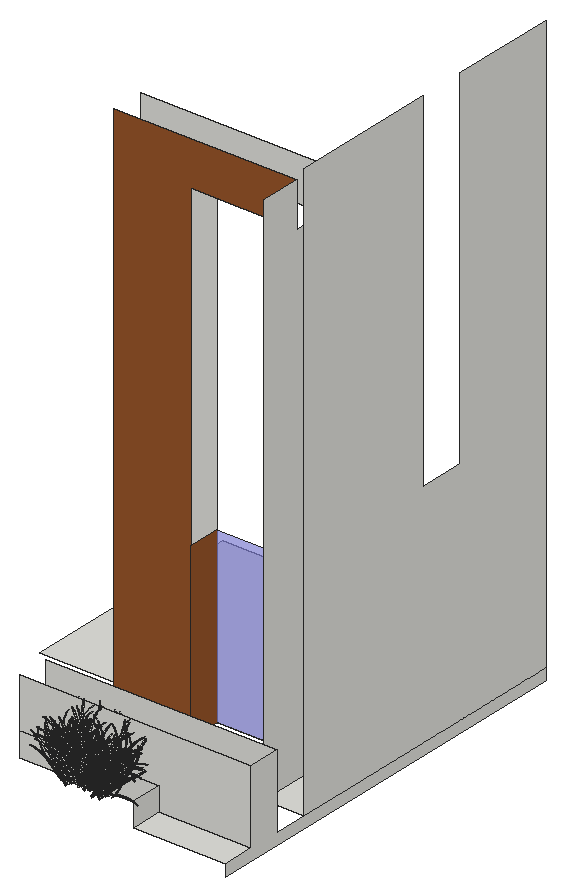
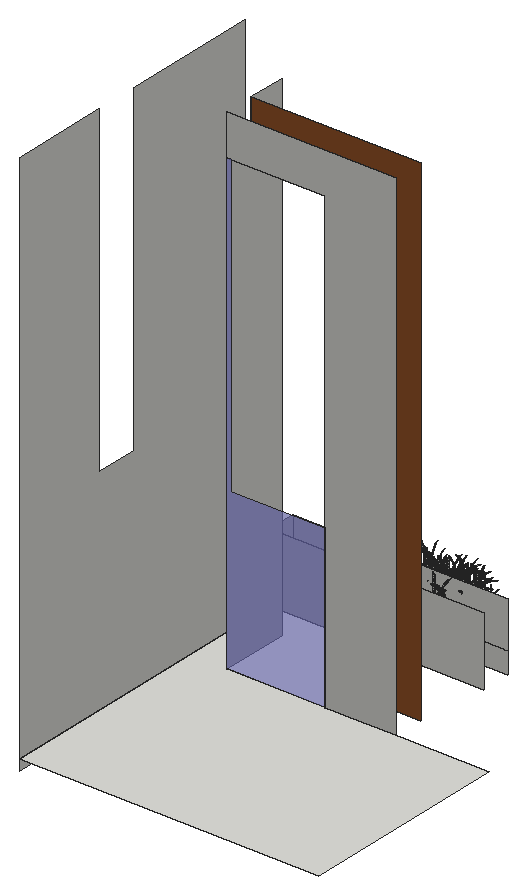
# SketchUp Ruby script. Lengths in inches.
U = 1.inch
M = Sketchup.active_model
def pt(a) = Geom::Point3d.new(a.map { |v| v * U })
def face(e, loops, mat)
  f = e.add_face(loops[0].map { |a| pt(a) })
  loops[1..].each { |l| e.add_face(l.map { |a| pt(a) }).erase! }
  f.material = f.back_material = mat if mat
  f
end
# faces: each face lists its corners as indices into pts; further lists are holes
def faces(e, pts, list, mat = nil) = list.each { |f| face(e, (f[0].is_a?(Array) ? f : [f]).map { |l| l.map { |i| pts[i] } }, mat) }
# xy, xz, yz: faces in a plane at the given z, y or x. An outline is a flat list of corners, or four numbers for a rectangle; further outlines are holes
def ring(l) = l.size == 4 ? [[l[0], l[1]], [l[2], l[1]], [l[2], l[3]], [l[0], l[3]]] : l.each_slice(2).to_a
def flat(e, list, mat, &to3) = list.each { |f| face(e, (f[0].is_a?(Array) ? f : [f]).map { |l| ring(l).map { |u, v| to3.(u, v) } }, mat) }
def xy(e, z, list, mat = nil) = flat(e, list, mat) { |x, y| [x, y, z] }
def xz(e, y, list, mat = nil) = flat(e, list, mat) { |x, z| [x, y, z] }
def yz(e, x, list, mat = nil) = flat(e, list, mat) { |y, z| [x, y, z] }
def lines(e, pts, list) = list.each { |a, b| e.add_line(pt(pts[a]), pt(pts[b])) }
# prism: a flat outline (further loops are holes) pulled along v
def prism(e, loops, v, mat = nil)
  f = face(e, loops, mat); d = Geom::Vector3d.new(v.map { |x| x * U })
  f.pushpull(f.normal.samedirection?(d) ? d.length : -d.length)
end
def box(e, o, s, mat = nil) = prism(e, [[o, [o[0] + s[0], o[1], o[2]], [o[0] + s[0], o[1] + s[1], o[2]], [o[0], o[1] + s[1], o[2]]]], [0, 0, s[2]], mat)
def at(x, y, z, deg = 0) = Geom::Transformation.translation(pt([x, y, z])) * Geom::Transformation.rotation(ORIGIN, Z_AXIS, deg.degrees)
def axes(o, x, y, z) = Geom::Transformation.new([*x, 0, *y, 0, *z, 0, *pt(o).to_a, 1])
def part(name) = M.definitions.add(name)
# library, detail: a bought-in or finely detailed component or shape, given as its bounding box
def library(name, o, s) = part(name).tap { |d| box(d.entities, o, s) }
def detail(e, o, s) = box(e.add_group.entities, o, s)
def put(e, d, t, mat = nil) = e.add_instance(d, t).tap { |i| i.material = mat if mat }
def group(e, t, mat = nil) = e.add_group.tap { |g| g.transformation = t; g.material = mat if mat }.entities
root = M.entities
M.materials.add("[Color I02]1").color = [153, 153, 255]
M.materials["[Color I02]1"].alpha = 0.68
M.materials.add("[Wood Cherry Original]").color = [152, 86, 42]
c1 = part("fur_instance\#8")
p = [[-0.25,1.49,0.03],[0.25,-1.49,-0.03],[0.44,-1.47,1.51],[-0.05,1.47,1.57],[0.65,-1.44,3.05],[0.16,1.45,3.11],
  [0.86,-1.42,4.59],[0.38,1.44,4.65],[1.1,-1.39,6.13],[0.62,1.43,6.18],[1.34,-1.35,7.66],[0.875,1.42,7.72],
  [1.6,-1.32,9.19],[1.14,1.41,9.25],[1.88,-1.28,10.72],[1.43,1.41,10.78],[2.18,-1.24,12.25],[1.73,1.41,12.3],
  [2.49,-1.19,13.77],[2.05,1.41,13.82],[2.83,-1.15,15.29],[2.4,1.41,15.34],[3.18,-1.09,16.8],[2.76,1.42,16.85],
  [3.56,-1.03,18.31],[3.14,1.43,18.35],[3.96,-0.97,19.81],[3.55,1.44,19.85],[4.38,-0.91,21.3],[3.99,1.46,21.35],
  [4.84,-0.83,22.78],[4.45,1.48,22.83],[5.32,-0.76,24.26],[4.93,1.51,24.31],[5.82,-0.67,25.73],[5.45,1.54,25.77],
  [6.36,-0.59,27.18],[6,1.57,27.23],[6.93,-0.49,28.625],[6.58,1.61,28.67],[7.54,-0.39,30.05],[7.19,1.66,30.1],
  [8.18,-0.28,31.47],[7.84,1.71,31.51],[8.85,-0.16,32.86],[8.53,1.77,32.9],[9.57,-0.04,34.24],[9.25,1.83,34.27],
  [10.32,0.09,35.59],[10.02,1.9,35.625],[11.12,0.23,36.92],[10.82,1.97,36.95],[11.95,0.38,38.22],[11.67,2.06,38.25],
  [12.84,0.54,39.49],[12.57,2.14,39.52],[13.76,0.71,40.73],[13.51,2.24,40.76],[14.73,0.89,41.93],[14.49,2.34,41.95],
  [15.75,1.08,43.09],[15.52,2.45,43.11],[16.82,1.28,44.2],[16.6,2.5625,44.23],[17.93,1.5,45.27],[17.73,2.68,45.29],
  [19.08,1.73,46.28],[18.9,2.81,46.3],[20.29,1.97,47.24],[20.125,2.93,47.26],[21.53,2.22,48.13],[21.39,3.0625,48.15],
  [22.82,2.5,48.96],[22.7,3.1875,48.98],[24.14,2.8125,49.72],[24.06,3.3,49.73],[25.48,3.27,50.41]]
faces(c1.entities,p,[[0,1,2,3],[3,2,4,5],[5,4,6,7],[7,6,8,9],[9,8,10,11],[11,10,12,13],[13,12,14,15],[15,14,16,17],
  [17,16,18,19],[19,18,20,21],[21,20,22,23],[23,22,24,25],[25,24,26,27],[27,26,28,29],[29,28,30,31],[31,30,32,33],
  [33,32,34,35],[35,34,36,37],[37,36,38,39],[39,38,40,41],[41,40,42,43],[43,42,44,45],[45,44,46,47],[47,46,48,49],
  [49,48,50,51],[51,50,52,53],[53,52,54,55],[55,54,56,57],[57,56,58,59],[59,58,60,61],[61,60,62,63],[63,62,64,65],
  [65,64,66,67],[67,66,68,69],[69,68,70,71],[71,70,72,73],[73,72,74,75],[75,74,76]])
xy(root,0,[[324.83,32.99,373.22,49.71],[352.27,84.18,352.27,122.8,204.07,122.8,204.07,242.8,373.22,242.8,373.22,84.18]])
xz(root,49.71,[[252.01,0,324.83,12.375],[324.83,0,373.22,0,373.22,38.6875,252.01,38.6875,252.01,12.375,324.83,12.375]])
xz(root,66.43,[[252.01,0,373.22,38.6875]])
xz(root,105.55,[[256.63,0,296.76,0,296.76,258.95,352.27,258.95,352.27,282.04,256.63,282.04]],"[Wood Cherry Original]")
xz(root,122.8,[[256.63,0,256.63,282.04,352.27,282.04,352.27,258.95,296.76,258.95,296.76,0]])
xz(root,122.8,[[296.76,0,352.27,0,352.27,258.95,349.59,258.95,349.59,90.8125,296.76,90.8125]],"[Color I02]1")
yz(root,296.76,[[105.55,0,122.8,90.8125]],"[Wood Cherry Original]")
yz(root,324.83,[[32.99,0,49.71,12.375]])
yz(root,352.27,[[84.18,0,84.18,282.04,105.55,282.04,105.55,258.95,122.8,258.95,122.8,0]])
yz(root,373.22,[[32.99,-6,242.8,-6,242.8,0,66.43,0,66.43,38.6875,49.71,38.6875,49.71,0,32.99,0],[84.18,0,242.8,0,242.8,304.31,186.78,304.31,186.78,120.43,162.34,120.43,162.34,304.31,84.18,304.31]])
put(root,c1,axes([297.07,29.66,14.5],[-0.37986,0.11496,-0.01734],[-0.11893,-0.25359,-0.04518],[-0.03923,-0.08677,0.40722]))
put(root,c1,axes([300.22,27.99,12.8],[-0.17462,0.20391,0.03429],[-0.27946,-0.10792,0.01354],[0.0209,-0.06883,0.33653]))
put(root,c1,axes([293.93,31.76,13.74],[-0.30043,-0.13979,-0.08203],[0.22786,-0.24984,0.08437],[-0.12286,-0.04065,0.38921]))
put(root,c1,axes([291.35,30.26,11.03],[0.27814,-0.07125,0.24103],[0.01578,0.25799,0.01434],[-0.24239,-0.02942,0.29163]))
put(root,c1,axes([309.31,30.78,9.9],[0.26005,-0.02253,-0.32035],[0.06182,0.2884,-0.05179],[0.3097,-0.0728,0.26576]))
put(root,c1,axes([306.62,31.4,9.98],[-0.12063,-0.20656,0.23753],[0.22477,-0.16177,-0.15489],[0.25439,0.01275,0.23669]))
put(root,c1,axes([300.89,28.39,13.19],[-0.00414,0.23821,0.05401],[-0.3412,-0.00346,0.09367],[0.08458,-0.09461,0.34384]))
put(root,c1,axes([292.09,29.77,9.76],[0.20353,-0.04601,0.26437],[-0.00599,0.23776,-0.01108],[-0.26313,-0.01442,0.2153]))
put(root,c1,axes([309.51,34.31,12.07],[-0.09639,-0.31824,0.12722],[0.35076,-0.08826,-0.26749],[0.27732,-0.04665,0.36362]))
put(root,c1,axes([298.73,28.3,13.26],[-0.08984,0.23712,0.03942],[-0.33625,-0.03634,-0.01926],[-0.01687,-0.08372,0.35457]))
put(root,c1,axes([302.43,31.45,14.3],[0.38172,-0.07813,-0.11304],[0.09285,0.27954,-0.03883],[0.10653,-0.06196,0.39986]))
put(root,c1,axes([302.73,28.04,12],[0.10021,0.21737,-0.04197],[-0.27272,0.07036,0.15178],[0.14611,-0.06349,0.29391]))
put(root,c1,axes([292.2,29.75,13.39],[-0.30752,0.22698,-0.0565],[-0.22359,-0.16067,-0.20167],[-0.1779,-0.12786,0.376]))
put(root,c1,axes([303.88,30.99,14.1],[0.39992,0.00155,-0.12267],[-0.00919,0.2918,0.01674],[0.11029,-0.07994,0.40704]))
put(root,c1,axes([295.86,30.04,13.95],[0.3361,0.0597,0.11647],[-0.14291,0.26481,-0.01688],[-0.12031,-0.07015,0.37628]))
put(root,c1,axes([314.07,32.9,10.36],[-0.31461,0.02837,0.40448],[-0.1367,-0.3405,0.01783],[0.37524,-0.14378,0.32832]))
put(root,c1,axes([298.375,28.95,14.06],[-0.23063,0.22567,0.03204],[-0.30414,-0.13521,-0.0359],[-0.0185,-0.09181,0.38884]))
put(root,c1,axes([290.27,32.23,9.95],[-0.02718,-0.26721,0.06111],[0.23487,-0.04018,0.2882],[-0.28708,0.02287,0.24209]))
put(root,c1,axes([305.03,31.13,9.43],[-0.06107,-0.20124,0.21197],[0.24192,-0.11583,-0.14036],[0.20685,0.04397,0.21399]))
put(root,c1,axes([294.54,31.76,12.14],[0.17245,-0.22481,0.15675],[0.27326,0.12505,0.06049],[-0.14508,0.02294,0.32196]))
put(root,c1,axes([295.24,33.11,14.17],[-0.1453,-0.26295,0.04416],[0.36594,-0.13308,0.10576],[-0.09136,-0.00185,0.39825]))
put(root,c1,axes([299.125,32.17,12.94],[-0.17065,-0.21754,0.08769],[0.31451,-0.14349,0.04448],[-0.00634,0.01342,0.35351]))
put(root,c1,axes([298.21,29.74,13.28],[0.32343,0.06667,0.01052],[-0.1253,0.24167,-0.02668],[-0.02751,-0.0389,0.35559]))
put(root,c1,axes([306.15,28.67,9.75],[-0.05331,0.21759,0.08334],[-0.21187,-0.0925,0.2518],[0.25313,-0.0595,0.21722]))
put(root,c1,axes([309.43,29.48,9.85],[0.01398,0.27039,0.10361],[-0.28188,-0.07693,0.31658],[0.30873,-0.11829,0.27013]))
put(root,c1,axes([295.78,30.16,12.95],[-0.33254,0.06855,-0.1047],[-0.04472,-0.24536,0.00177],[-0.10933,-0.03618,0.34634]))
put(root,c1,axes([299.96,30.99,13.19],[0.3311,-0.11143,-0.00818],[0.12332,0.23349,-0.09764],[0.03307,0.00434,0.3504]))
put(root,c1,axes([300.49,31.6,11.78],[0.12505,-0.22688,0.10637],[0.2992,0.06356,-0.10951],[0.05567,0.04516,0.30083]))
put(root,c1,axes([295.53,30.05,14.23],[0.26883,0.15362,0.11698],[-0.26881,0.22996,-0.03987],[-0.11858,-0.08853,0.38915]))
put(root,c1,axes([297.49,30.97,13.59],[-0.33593,-0.07204,-0.02348],[0.12579,-0.25592,0.09942],[-0.06598,0.00622,0.35973]))
put(root,c1,axes([300.72,29.6875,12.73],[0.31871,0.03853,-0.0833],[-0.07703,0.23988,-0.04321],[0.06207,-0.01348,0.32903]))
put(root,c1,axes([308.82,35.61,14.78],[0.22107,-0.31645,-0.08819],[0.39347,0.17405,-0.22486],[0.22281,-0.06522,0.45604]))
put(root,c1,axes([292.26,33,12.65],[-0.21857,-0.2084,-0.04599],[0.27515,-0.19846,0.18316],[-0.1798,0.00438,0.35795]))
put(root,c1,axes([299.6875,29.61,13.07],[0.27771,0.12403,-0.02683],[-0.1961,0.21075,-0.00493],[0.0103,-0.04126,0.34765]))
put(root,c1,axes([295.9375,29.46,12.93],[-0.25046,0.19218,-0.07567],[-0.21771,-0.16026,-0.07349],[-0.11089,-0.04968,0.34288]))
put(root,c1,axes([292.76,30.24,14.75],[-0.06283,0.2928,0.10996],[-0.40135,0.05052,-0.19489],[-0.19008,-0.13661,0.40174]))
put(root,c1,axes([305.98,30.41,12.04],[-0.21613,0.17279,0.19106],[-0.21553,-0.21071,0.16457],[0.23814,-0.07365,0.30654]))
put(root,c1,axes([299.64,33.21,13.75],[-0.22461,-0.21558,0.09909],[0.31674,-0.18353,0.03994],[0.01515,0.01113,0.38383]))
put(root,c1,axes([304.03,29.54,11.83],[-0.20447,0.18723,0.09128],[-0.23214,-0.16193,0.13811],[0.15272,-0.0447,0.31258]))
put(root,c1,axes([301.73,29.38,12.42],[0.25056,0.13748,-0.09261],[-0.20183,0.19585,0.01597],[0.07293,-0.02461,0.32493]))
put(root,c1,axes([293.94,30.14,13.9],[-0.26766,0.23648,-0.03819],[-0.2782,-0.15147,-0.11955],[-0.12042,-0.0899,0.39518]))
put(root,c1,axes([295.06,30.1875,12.98],[-0.31485,0.13604,-0.10356],[-0.13695,-0.22237,-0.02752],[-0.11187,-0.03702,0.3544]))
put(root,c1,axes([293.16,32.5625,11.3],[-0.03678,-0.25397,0.12997],[0.29931,-0.02143,0.19004],[-0.19333,0.05707,0.28615]))
put(root,c1,axes([304.64,31.96,13.24],[-0.36491,-0.01389,0.1859],[0.03737,-0.29294,0.04841],[0.16886,-0.0262,0.36677]))
put(root,c1,axes([296.76,30.3125,12.78],[-0.31334,0.10011,-0.09501],[-0.10112,-0.22757,0.02464],[-0.08992,-0.01108,0.3359]))
put(root,c1,axes([291.74,31.81,9.48],[0.14355,-0.1766,0.25684],[0.18766,0.16788,0.08409],[-0.24795,0.05471,0.22422]))
put(root,c1,axes([295.6,32.125,12.85],[-0.2833,-0.13793,-0.02305],[0.18987,-0.22311,0.16973],[-0.12695,0.04004,0.33147]))
put(root,c1,axes([291.51,30.93,13.19],[0.25521,0.1512,0.17452],[-0.25665,0.25153,-0.10558],[-0.20333,-0.07415,0.37359]))
put(root,c1,axes([298.13,31.5625,11.92],[-0.26729,-0.12063,0.06749],[0.18715,-0.19794,0.13627],[-0.03388,0.05903,0.30001]))
put(root,c1,axes([302.29,30.11,13.34],[0.22509,0.19991,-0.07599],[-0.27838,0.17319,0.07803],[0.09708,-0.05646,0.36438]))
put(root,c1,axes([304.44,30.18,12.87],[-0.10789,0.25373,0.07285],[-0.32713,-0.09482,0.17189],[0.17322,-0.07527,0.34846]))
put(root,c1,axes([301.9375,33.34,12.41],[-0.18573,-0.21093,0.17304],[0.30858,-0.16641,-0.00938],[0.0929,0.03699,0.33971]))
put(root,c1,axes([301.17,33.54,12.34],[0.02005,-0.26344,0.15335],[0.36284,-0.01782,-0.07584],[0.06238,0.05061,0.33711]))
put(root,c1,axes([302.27,33.05,14.28],[0.3894,-0.10534,-0.06303],[0.1122,0.28119,-0.09735],[0.07672,-0.01666,0.40666]))
put(root,c1,axes([304.9375,32.15,11.95],[0.31108,-0.11547,-0.14728],[0.08809,0.24884,-0.19208],[0.19555,0.02546,0.30249]))
put(root,c1,axes([310.28,36.01,13.41],[0.26375,-0.26825,-0.16948],[0.29485,0.23881,-0.27394],[0.30159,-0.05073,0.39544]))
put(root,c1,axes([305.46,33.45,11.4],[0.25076,-0.21435,-0.05395],[0.21574,0.18121,-0.2417],[0.20008,0.02605,0.30949]))
put(root,c1,axes([307.5,33.67,12.11],[0.30932,-0.16941,-0.1706],[0.16282,0.26082,-0.21532],[0.24459,-0.00639,0.3404]))
put(root,c1,axes([296.91,34.89,14.07],[-0.1186,-0.27751,0.08841],[0.38874,-0.1102,0.0715],[-0.0532,0.01296,0.40459]))
put(root,c1,axes([306.88,34.04,11.42],[-0.17025,-0.23312,0.23887],[0.30544,-0.18356,-0.10713],[0.2115,0.02754,0.32717]))
put(root,c1,axes([303.75,30.85,11.85],[-0.31518,0.08138,0.11458],[-0.07485,-0.24165,0.11876],[0.13173,-0.00126,0.31832]))
put(root,c1,axes([302.64,34.5625,16.18],[0.42095,-0.14725,-0.10442],[0.17691,0.30585,-0.08745],[0.1162,-0.05293,0.46349]))
put(root,c1,axes([292.29,31.73,12.13],[-0.32982,0.0527,-0.18032],[-0.01849,-0.26967,0.0269],[-0.1831,-0.01848,0.34164]))
put(root,c1,axes([294.35,32.48,11.32],[-0.17974,-0.20388,0.06604],[0.25023,-0.12836,0.21159],[-0.15875,0.07631,0.27776]))
put(root,c1,axes([288.31,31.25,10.58],[0.14971,0.15077,0.26268],[-0.21096,0.2535,-0.19987],[-0.32252,-0.06234,0.26598]))
put(root,c1,axes([297.09,29.33,12.93],[0.00143,0.24353,-0.03417],[-0.32321,0.03016,-0.09258],[-0.09858,-0.02214,0.33211]))
put(root,c1,axes([300.8,30.81,14.04],[0.32079,0.12524,-0.10886],[-0.18999,0.24738,0.00297],[0.08451,-0.02851,0.37652]))
put(root,c1,axes([287.89,32.19,11.4],[0.25708,0.10485,0.25987],[-0.20499,0.28763,-0.11391],[-0.27939,-0.07246,0.33941]))
put(root,c1,axes([295.05,32.47,13.86],[0.38017,-0.03428,0.09673],[0.00663,0.28506,-0.0591],[-0.10384,-0.01279,0.3879]))
put(root,c1,axes([304.9,35.46,13.89],[-0.21678,-0.25794,0.18892],[0.34901,-0.19506,-0.09005],[0.16707,-0.0016,0.40371]))
put(root,c1,axes([297.7,30.01,13.23],[-0.01029,0.24957,-0.01761],[-0.34619,0.0186,-0.02439],[-0.03281,-0.04143,0.35542]))
put(root,c1,axes([299.64,31.97,12.16],[-0.30501,-0.08008,0.0968],[0.14614,-0.2274,0.12372],[0.02756,0.05561,0.31043]))
put(root,c1,axes([297.65,32.28,14.4375],[-0.38282,0.09711,-0.02143],[-0.09773,-0.2685,0.02287],[-0.02447,-0.04231,0.40465]))
put(root,c1,axes([294.07,30.88,10.86],[0.25741,0.03344,0.16681],[-0.0417,0.2339,-0.12911],[-0.1963,0.02845,0.25979]))
put(root,c1,axes([299.35,30.33,13.14],[-0.29118,0.15292,-0.03089],[-0.18473,-0.19959,0.08971],[0.01345,0.00988,0.34087]))
put(root,c1,axes([296.21,30.16,13.16],[0.14937,0.21705,0.01001],[-0.30573,0.14011,-0.10341],[-0.10379,-0.02331,0.34963]))
put(root,c1,axes([299.28,30.3,13.45],[0.09139,0.24124,-0.02708],[-0.34395,0.08755,0.00024],[-0.00171,-0.03839,0.36389]))
put(root,c1,axes([292,30.13,11.09],[0.06312,0.2347,0.05533],[-0.26357,0.11274,-0.22829],[-0.2358,-0.02862,0.28371]))
put(root,c1,axes([301.01,29.86,12.8],[0.02445,0.24426,-0.06773],[-0.33257,0.03724,0.06724],[0.06313,-0.01371,0.33464]))
put(root,c1,axes([301.4375,33.59,16.1875],[0.44361,0.00954,-0.12956],[-0.03541,0.33069,-0.02892],[0.11325,-0.05159,0.45172]))
put(root,c1,axes([298.8125,30.33,12.92],[-0.24792,0.18255,-0.06135],[-0.23021,-0.1655,0.06985],[-0.00599,0.01269,0.33425]))
put(root,c1,axes([292.85,31.49,13.32],[0.22087,0.18128,0.12698],[-0.26546,0.22192,-0.14635],[-0.19746,-0.04494,0.3589]))
put(root,c1,axes([301.2,30.7,12.46],[-0.2311,0.19122,-0.01481],[-0.24074,-0.15447,0.09263],[0.04816,-0.00374,0.33273]))
put(root,c1,axes([307.89,32.19,14.26],[-0.10311,0.30987,0.12078],[-0.41871,-0.10394,0.20078],[0.20991,-0.12435,0.43231]))
put(root,c1,axes([299.71,32.49,11.62],[-0.31244,-0.05998,0.08505],[0.11859,-0.23055,0.12985],[0.02723,0.05495,0.30674]))
put(root,c1,axes([288.9375,33.78,11.8],[0.31888,-0.08776,0.27392],[0.0591,0.29525,-0.01943],[-0.27072,0.00273,0.33496]))
put(root,c1,axes([290.05,34.25,10.97],[0.26388,-0.16586,0.25638],[0.17817,0.23606,0.02465],[-0.23968,0.03474,0.31721]))
put(root,c1,axes([303.36,31.49,11.12],[0.28654,0.0293,-0.18535],[-0.09478,0.23872,-0.10787],[0.14833,0.04775,0.26999]))
put(root,c1,axes([306.97,32.19,13.47],[0.21529,0.26732,-0.1015],[-0.33179,0.15897,0.18881],[0.1989,-0.08642,0.4001]))
put(root,c1,axes([296.45,32.43,13.07],[0.34376,0.06003,0.02841],[-0.1102,0.26073,-0.0988],[-0.0664,0.00626,0.36202]))
put(root,c1,axes([307.04,31.4,11.7],[-0.10758,0.27316,0.04345],[-0.30064,-0.09702,0.25634],[0.24342,-0.04095,0.31917]))
put(root,c1,axes([294.3125,31.78,13.16],[-0.28482,0.16744,-0.17926],[-0.17967,-0.21914,-0.02481],[-0.1723,0.0042,0.34303]))
put(root,c1,axes([297.99,32.49,12.83],[0.3546,-0.04207,0.0418],[0.03679,0.24974,-0.16079],[-0.03701,0.06449,0.32778]))
put(root,c1,axes([303.89,30.28,11.28],[-0.00719,0.23917,-0.12291],[-0.2843,0.03205,0.17385],[0.17201,0.0224,0.26607]))
put(root,c1,axes([310.13,32.77,9.65],[-0.23743,0.1703,0.23472],[-0.15105,-0.25518,0.23763],[0.31546,-0.02981,0.27622]))
put(root,c1,axes([292.56,33.74,13.97],[-0.37552,0.02978,-0.18444],[-0.00274,-0.30609,0.08192],[-0.19214,0.00468,0.38253]))
put(root,c1,axes([301.625,32.89,11.47],[0.32327,-0.10712,-0.01749],[0.09339,0.2108,-0.21888],[0.08265,0.08899,0.27927]))
put(root,c1,axes([289.88,32.2,9.47],[0.22299,0.08012,0.23253],[-0.07774,0.25772,-0.18032],[-0.28674,0.02285,0.2418]))
put(root,c1,axes([299.68,31.02,13.39],[0.09517,0.24549,-0.09781],[-0.34506,0.0918,0.01689],[0.0335,0.00439,0.35498]))
put(root,c1,axes([298.21,35.625,12.82],[0.21798,-0.24571,0.14926],[0.32986,0.13334,-0.10586],[-0.00426,0.0705,0.36176]))
put(root,c1,axes([297.91,36.18,12.93],[0.12837,-0.2754,0.18421],[0.3803,0.07387,-0.03249],[-0.04167,0.07261,0.36905]))
put(root,c1,axes([292.99,32.01,10.625],[-0.21375,0.16044,-0.2188],[-0.17312,-0.19073,-0.04043],[-0.20706,0.03001,0.27404]))
put(root,c1,axes([296.8,36.26,12.95],[0.11216,-0.27982,0.18642],[0.38756,0.06205,-0.02451],[-0.04189,0.07299,0.37096]))
put(root,c1,axes([300.57,32.22,11.33],[-0.32555,0.01552,0.05629],[0.02551,-0.21913,0.2004],[0.03956,0.09625,0.26535]))
put(root,c1,axes([303.87,34.79,9.58],[-0.07713,-0.20181,0.27533],[0.31715,-0.12915,-0.06147],[0.15566,0.11006,0.24058]))
put(root,c1,axes([294.44,31.52,11.55],[0.10989,0.22592,-0.04424],[-0.2903,0.10013,-0.15522],[-0.13937,0.02203,0.30928]))
put(root,c1,axes([302.81,32.85,15.3125],[0.10532,0.30402,-0.04355],[-0.41529,0.08818,0.12286],[0.11618,-0.06757,0.43608]))
put(root,c1,axes([293.17,34.71,15.125],[-0.41497,0.11282,-0.12938],[-0.10014,-0.30383,0.01576],[-0.1302,-0.02924,0.43863]))
put(root,c1,axes([296.16,32.57,11.97],[0.30429,0.09538,0.01629],[-0.13866,0.22954,-0.16183],[-0.09588,0.05048,0.31741]))
put(root,c1,axes([292.96,34.11,9.71],[-0.28109,-0.11553,-0.06299],[0.09114,-0.20051,0.26985],[-0.19429,0.11376,0.23386]))
put(root,c1,axes([301.5,31.45,11.39],[-0.09337,0.22828,-0.11476],[-0.30505,-0.0402,0.09688],[0.05476,0.04443,0.29594]))
put(root,c1,axes([299.04,34.23,13.18],[0.3826,-0.06128,0.01902],[0.05373,0.26621,-0.17779],[-0.00416,0.06889,0.3535]))
put(root,c1,axes([296.6875,32.12,11.73],[-0.22053,0.18022,-0.15283],[-0.23513,-0.15794,0.03506],[-0.09243,0.04867,0.306]))
put(root,c1,axes([294.78,34.97,10.76],[0.2625,-0.14738,0.21205],[0.21669,0.19878,-0.09487],[-0.13116,0.09754,0.29312]))
put(root,c1,axes([295.42,33.2,10.49],[0.31269,0.01357,0.09328],[-0.00239,0.22692,-0.19194],[-0.12049,0.0896,0.26927]))
put(root,c1,axes([307.39,32.0625,9.94],[0.01192,0.2682,-0.15387],[-0.26672,0.05898,0.25379],[0.26625,0.01334,0.24773]))
put(root,c1,axes([294.62,33.49,10.86],[0.31025,0.02136,0.12942],[-0.00842,0.24175,-0.18196],[-0.15992,0.07687,0.2798]))
put(root,c1,axes([298.14,34.6875,10.125],[-0.03498,-0.20006,0.26264],[0.33857,-0.02028,0.05275],[-0.05072,0.15008,0.22962]))
put(root,c1,axes([304.75,33.74,11.91],[-0.34714,0.09005,0.13903],[-0.04585,-0.2641,0.20633],[0.17209,0.0554,0.31324]))
put(root,c1,axes([303.93,35.28,10.24],[0.30429,-0.17714,0.00045],[0.15067,0.17535,-0.29348],[0.16193,0.1145,0.25028]))
put(root,c1,axes([301.15,35.4,9.74],[0.02171,-0.21225,0.26978],[0.35113,-0.03257,-0.06302],[0.05505,0.14594,0.23778]))
put(root,c1,axes([304.93,33.43,14.19],[0.16792,0.28009,-0.14825],[-0.36004,0.14978,0.14596],[0.18288,-0.02838,0.39722]))
put(root,c1,axes([295.57,33.97,11.49],[0.33335,-0.01288,0.12248],[0.03512,0.24333,-0.19321],[-0.12916,0.09605,0.28864]))
put(root,c1,axes([298.59,34.16,14.93],[-0.36467,0.17722,-0.05568],[-0.21281,-0.2513,0.10179],[-0.00748,0.01584,0.41713]))
put(root,c1,axes([297.71,32.1,12.31],[0.07759,0.23448,-0.13461],[-0.3281,0.06649,-0.08615],[-0.06621,0.05797,0.31394]))
put(root,c1,axes([297.97,32.45,11.12],[0.26871,0.1121,-0.09185],[-0.17857,0.18234,-0.18441],[-0.04158,0.10221,0.26229]))
put(root,c1,axes([291.68,33.52,9.99],[-0.2282,0.09889,-0.27706],[-0.15507,-0.22815,0.06699],[-0.23524,0.08977,0.23863]))
put(root,c1,axes([303.21,36.85,11.17],[-0.22074,-0.19332,0.24763],[0.32228,-0.19488,0.06048],[0.09595,0.1033,0.32421]))
put(root,c1,axes([301.02,33.47,9.91],[-0.32142,0.01588,0.07582],[0.04323,-0.19732,0.24388],[0.05075,0.13454,0.2192]))
put(root,c1,axes([291.42,35.39,9.9],[0.25074,-0.08755,0.28619],[0.14655,0.24668,-0.09015],[-0.24763,0.0945,0.2512]))
put(root,c1,axes([301.02,34.29,13.54],[-0.37668,0.11666,0.0198],[-0.11531,-0.26137,0.1844],[0.06763,0.05486,0.36544]))
put(root,c1,axes([299.37,33.28,14.04],[-0.08791,0.28558,-0.09756],[-0.38541,-0.03903,0.04808],[0.01542,0.01133,0.39076]))
put(root,c1,axes([291.32,33.33,11.09],[-0.13915,0.24729,-0.20336],[-0.27037,-0.1215,-0.13837],[-0.2289,0.03317,0.30295]))
put(root,c1,axes([297.18,33.7,9.77],[-0.30471,0.02079,-0.10877],[-0.06538,-0.19372,0.22972],[-0.09578,0.13621,0.21711]))
put(root,c1,axes([307.42,34.21,10.3],[-0.29712,0.14734,0.1685],[-0.08067,-0.24572,0.26461],[0.25524,0.05426,0.26405]))
put(root,c1,axes([306.58,34.3,12.69],[0.2149,0.22877,-0.24278],[-0.27792,0.213,0.13148],[0.24582,-0.00643,0.34211]))
put(root,c1,axes([297.23,35.37,10.27],[0.21532,-0.16466,0.23481],[0.27912,0.12752,-0.1478],[-0.05253,0.15544,0.23782]))
put(root,c1,axes([304.37,34.36,11.59],[-0.32789,0.1435,0.09153],[-0.1181,-0.23778,0.2301],[0.17128,0.05514,0.31177]))
put(root,c1,axes([291.21,38.76,11.93],[0.03426,-0.30148,0.23803],[0.38836,0.04526,0.14837],[-0.20088,0.09657,0.35147]))
put(root,c1,axes([303.36,33.71,10.27],[-0.31347,0.1074,0.08336],[-0.04707,-0.20642,0.26099],[0.15117,0.10689,0.23365]))
put(root,c1,axes([304.01,33.1,10.39],[-0.22722,0.20575,-0.01496],[-0.18573,-0.12856,0.27335],[0.19083,0.07929,0.23211]))
put(root,c1,axes([300.94,34,11.25],[0.31948,0.06732,-0.13282],[-0.14912,0.22743,-0.18129],[0.04271,0.10392,0.2865]))
put(root,c1,axes([296.73,35.09,15.26],[0.34747,0.16946,-0.03102],[-0.25995,0.27004,-0.11737],[-0.05681,0.01384,0.43198]))
put(root,c1,axes([308.42,34.29,9.73],[-0.16741,0.26625,0.03865],[-0.23369,-0.12855,0.31721],[0.28667,0.01437,0.26672]))
put(root,c1,axes([290.1,35.47,14.55],[0.26115,0.22486,0.10659],[-0.3089,0.25028,-0.19615],[-0.22421,-0.02263,0.41834]))
put(root,c1,axes([294.53,33.1,10.75],[-0.0094,0.23776,-0.17948],[-0.3052,-0.02188,-0.12668],[-0.15733,0.07563,0.27528]))
put(root,c1,axes([289.83,37.49,11.28],[0.3275,-0.1168,0.26372],[0.15078,0.28145,-0.07889],[-0.23114,0.06823,0.34212]))
put(root,c1,axes([302.13,36.55,14.42],[0.42486,0.00795,-0.14048],[-0.06464,0.32048,-0.15173],[0.11085,0.04413,0.40535]))
put(root,c1,axes([302.29,34.15,12.1875],[-0.3135,0.16987,0.01114],[-0.167,-0.20326,0.24037],[0.13137,0.078,0.30476]))
put(root,c1,axes([295.39,36.1875,10.66],[0.33995,-0.08561,0.14528],[0.13056,0.23485,-0.18927],[-0.09324,0.11245,0.30268]))
put(root,c1,axes([293.92,34.72,11.03],[-0.27426,0.12888,-0.22321],[-0.18187,-0.22273,0.07892],[-0.16956,0.08151,0.29667]))
put(root,c1,axes([301.71,37.94,12.88],[0.34147,-0.21227,0.0692],[0.24226,0.20372,-0.26431],[0.10284,0.11072,0.34749]))
put(root,c1,axes([306.35,36.45,11.83],[0.37826,0.00458,-0.22144],[-0.08147,0.30831,-0.16295],[0.19016,0.06122,0.34614]))
put(root,c1,axes([304.49,36.6,11.29],[0.38407,-0.04972,-0.14005],[-0.0124,0.28223,-0.21944],[0.14212,0.08438,0.32969]))
put(root,c1,axes([306.7,37.35,10.33],[-0.2882,-0.08649,0.31541],[0.20824,-0.28093,0.1026],[0.2312,0.09606,0.28122]))
put(root,c1,axes([312.66,39.45,12.56],[-0.42715,-0.02419,0.32817],[0.06651,-0.38387,0.08793],[0.30249,-0.00791,0.42097]))
put(root,c1,axes([291.51,35.48,10.39],[0.29431,0.04362,0.2094],[0.00668,0.26171,-0.22058],[-0.251,0.09579,0.25462]))
put(root,c1,axes([300.52,36.84,12.89],[-0.41299,0.03386,0.04001],[-0.00291,-0.29245,0.18761],[0.03366,0.06791,0.37907]))
put(root,c1,axes([310.5,40.86,11.73],[-0.13778,-0.29005,0.35264],[0.36274,-0.21506,-0.17875],[0.32168,0.06838,0.33279]))
put(root,c1,axes([299.37,37.77,12.49],[0.33122,-0.18689,0.15289],[0.2535,0.20157,-0.21508],[-0.00144,0.13013,0.33652]))
put(root,c1,axes([308.93,34.72,9.85],[-0.00687,0.30102,-0.15108],[-0.29585,0.04507,0.29223],[0.29511,0.01479,0.27458]))
put(root,c1,axes([303.06,37.22,13.75],[-0.42743,0.07152,0.09854],[-0.04242,-0.31234,0.18166],[0.11079,0.04411,0.40514]))
put(root,c1,axes([307.03,41.19,12.63],[0.2599,-0.31873,0.06706],[0.35593,0.1475,-0.30589],[0.2166,0.06973,0.39426]))
put(root,c1,axes([302.15,33.85,11.16],[0.07213,0.22522,-0.22426],[-0.3401,0.09466,0.03435],[0.0854,0.09194,0.28855]))
put(root,c1,axes([295.42,34.38,11.47],[0.26352,0.16628,-0.05182],[-0.2153,0.18316,-0.22638],[-0.13112,0.09751,0.29304]))
put(root,c1,axes([298.42,37.23,13.28],[-0.42137,0.02708,0.0056],[-0.00179,-0.2967,0.19494],[-0.00454,0.07514,0.38554]))
put(root,c1,axes([295.73,34.89,12.68],[-0.22933,0.22711,-0.17211],[-0.30435,-0.15593,0.05487],[-0.07483,0.06553,0.35485]))
put(root,c1,axes([302.41,35.34,11.77],[-0.35266,0.13842,0.00001],[-0.13312,-0.22585,0.24598],[0.09259,0.09969,0.31285]))
put(root,c1,axes([302.54,36.24,10.17],[-0.34668,0.00002,0.16605],[0.10374,-0.23905,0.24417],[0.11321,0.13888,0.25286]))
put(root,c1,axes([296.6,36.59,11.17],[-0.3813,0.02071,-0.04148],[-0.01778,-0.25239,0.24019],[-0.04919,0.12092,0.31033]))
put(root,c1,axes([299.71,33.95,9.75],[-0.12599,0.1857,-0.23333],[-0.30463,-0.05364,0.10641],[0.00132,0.14289,0.22018]))
put(root,c1,axes([291.79,36.76,14.23],[-0.33372,0.20578,-0.21383],[-0.24038,-0.25468,0.00327],[-0.18466,0.0292,0.40979]))
put(root,c1,axes([295.15,35.625,15.47],[0.07852,0.31662,-0.09055],[-0.4353,0.08503,-0.08758],[-0.08136,0.00767,0.44358]))
put(root,c1,axes([288.92,37.31,11.92],[0.36947,0.05041,0.18865],[-0.04561,0.31057,-0.21258],[-0.23866,0.07045,0.35325]))
put(root,c1,axes([292.39,35.6,14.32],[0.01367,0.31876,-0.11898],[-0.40177,0.02856,-0.17186],[-0.1805,0.02854,0.40055]))
put(root,c1,axes([297.68,38.93,10.55],[0.07836,-0.23298,0.31495],[0.3945,0.04674,-0.03186],[-0.05994,0.17735,0.27135]))
put(root,c1,axes([294.41,34.6875,9.85],[0.21397,0.18598,-0.12116],[-0.23548,0.11646,-0.24718],[-0.15132,0.13358,0.23391]))
put(root,c1,axes([292.83,38.43,10],[0.26548,-0.13957,0.28848],[0.25342,0.21117,-0.13271],[-0.17456,0.15409,0.26982]))
put(root,c1,axes([305.96,39.49,10.09],[-0.25932,-0.14611,0.33128],[0.29947,-0.25143,0.08652],[0.18892,0.13358,0.29199]))
put(root,c1,axes([304.72,41.42,12.91],[0.35972,-0.25581,0.03582],[0.27505,0.22046,-0.30467],[0.16747,0.09944,0.38851]))
put(root,c1,axes([302.55,40.09,9.99],[-0.09732,-0.23155,0.33127],[0.39501,-0.13642,-0.02153],[0.12728,0.15613,0.28427]))
put(root,c1,axes([305.14,41.64,12.39],[-0.25869,-0.23017,0.30476],[0.36959,-0.24537,0.02287],[0.16684,0.09906,0.38705]))
put(root,c1,axes([306.95,35.87,10.84],[-0.11682,0.297,-0.11687],[-0.29865,-0.02915,0.30513],[0.26586,0.05652,0.27504]))
put(root,c1,axes([291.64,40,10.8125],[0.06295,-0.25616,0.33273],[0.38873,0.09023,0.07333],[-0.18729,0.16533,0.2895]))
put(root,c1,axes([292.7,35.6,10.28],[0.25121,0.18786,-0.0324],[-0.19191,0.16123,-0.29466],[-0.20785,0.1217,0.25018]))
put(root,c1,axes([300.36,36.91,15.48],[0.07458,0.32412,-0.12197],[-0.45103,0.08366,0.03458],[0.04279,0.00561,0.45337]))
put(root,c1,axes([291.96,39.58,14.48],[0.44422,0.0077,0.13813],[-0.02634,0.34217,-0.1757],[-0.16565,0.05224,0.43251]))
put(root,c1,axes([295.34,36.37,11.39],[-0.26525,0.17982,-0.21681],[-0.26655,-0.18517,0.11704],[-0.09629,0.11611,0.31256]))
put(root,c1,axes([298.34,36.66,10.54],[0.36323,0.03464,-0.08776],[-0.09991,0.21815,-0.27961],[0.00151,0.16329,0.25161]))
put(root,c1,axes([296.57,37.88,16.47],[-0.32829,0.27565,-0.11166],[-0.35147,-0.21756,0.07209],[-0.03602,0.01858,0.47629]))
put(root,c1,axes([306.02,36.02,9.94],[-0.05641,0.27329,-0.21756],[-0.32994,0.04346,0.22398],[0.21766,0.09043,0.26474]))
put(root,c1,axes([290.28,38,12.17],[0.30671,0.1858,0.0706],[-0.20831,0.25234,-0.27412],[-0.23769,0.07017,0.35181]))
put(root,c1,axes([290.9,37.84,10.74],[-0.2561,0.14005,-0.3145],[-0.23719,-0.23476,0.09074],[-0.22951,0.13438,0.27625]))
put(root,c1,axes([307.5625,38.53,14.88],[0.13241,0.34234,-0.18022],[-0.44893,0.13613,0.1561],[0.19033,-0.00183,0.45992]))
put(root,c1,axes([306.74,39.9375,10.8],[-0.37717,0.05337,0.25249],[0.05977,-0.31116,0.2513],[0.24832,0.10317,0.30203]))
put(root,c1,axes([295.35,38.03,12.52],[-0.33315,0.15868,-0.21082],[-0.23691,-0.23143,0.16521],[-0.10467,0.12623,0.33978]))
put(root,c1,axes([299.99,38.14,13.44],[-0.27152,0.26137,-0.12674],[-0.33932,-0.16629,0.15711],[0.03541,0.07146,0.39888]))
put(root,c1,axes([299.84,38.33,11.27],[0.33259,0.12189,-0.18697],[-0.23311,0.24454,-0.17908],[0.0492,0.11972,0.33005]))
put(root,c1,axes([295.4375,39.05,11.76],[-0.38715,0.08937,-0.158],[-0.13683,-0.26731,0.21776],[-0.10514,0.12679,0.3413]))
put(root,c1,axes([299.06,37.66,10.33],[-0.35896,0.1108,-0.10677],[-0.15016,-0.19943,0.28324],[0.00156,0.16866,0.25988]))
put(root,c1,axes([297.58,40.57,12.68],[-0.44662,-0.00971,0.04606],[0.05707,-0.29657,0.28112],[-0.00155,0.14048,0.36328]))
put(root,c1,axes([302.8,38.62,15.53],[0.16646,0.30885,-0.21955],[-0.43845,0.16434,0.05212],[0.12097,0.04816,0.44236]))
put(root,c1,axes([300.46,42.39,12.08],[-0.38591,-0.13282,0.20885],[0.25754,-0.28245,0.20939],[0.0562,0.13676,0.37701]))
put(root,c1,axes([303.4,37.26,10.29],[0.04662,0.22984,-0.30488],[-0.37713,0.10095,0.05657],[0.11889,0.14584,0.26553]))
put(root,c1,axes([294.25,39.35,17.55],[-0.08012,0.37488,-0.1312],[-0.50083,-0.02806,-0.06043],[-0.09329,0.0088,0.50864]))
put(root,c1,axes([296.5625,38.25,12.96],[0.29382,0.19611,-0.17071],[-0.30616,0.20197,-0.21043],[-0.05468,0.13443,0.34498]))
put(root,c1,axes([294.74,39.32,14.18],[0.30577,0.22958,-0.10031],[-0.33138,0.23138,-0.18874],[-0.08854,0.07753,0.41986]))
put(root,c1,axes([289.74,41.46,14.44],[0.43688,0.1148,0.08342],[-0.16541,0.34046,-0.21929],[-0.17389,0.05484,0.45404]))
put(root,c1,axes([294.96,40.24,16.79],[0.20675,0.32246,-0.09697],[-0.45736,0.17887,-0.10156],[-0.06571,0.016,0.49965]))
put(root,c1,axes([305.84,40.13,14.89],[-0.21963,0.34261,-0.06934],[-0.42375,-0.12981,0.22563],[0.16111,0.02613,0.4594]))
put(root,c1,axes([299.67,40.18,9.82],[0.40735,0.0263,-0.08168],[-0.09051,0.24325,-0.31417],[0.00167,0.18087,0.2787]))
put(root,c1,axes([303.34,40.92,10.67],[0.40714,0.00133,-0.19668],[-0.12398,0.28115,-0.28623],[0.13315,0.16334,0.29739]))
put(root,c1,axes([293.23,40.27,9.92],[-0.36993,0.07933,-0.20113],[-0.16637,-0.24085,0.26265],[-0.12466,0.17728,0.28258]))
put(root,c1,axes([303.91,40.14,16.58],[-0.04858,0.37725,-0.15234],[-0.48912,0.00642,0.18942],[0.16591,0.02691,0.4731]))
put(root,c1,axes([295.22,39.78,15.42],[-0.06391,0.33969,-0.21918],[-0.46754,-0.03126,-0.04471],[-0.09267,0.08114,0.4394]))
put(root,c1,axes([299.3125,40.23,11.31],[-0.27908,0.23344,-0.20203],[-0.32938,-0.16264,0.18381],[-0.00149,0.13469,0.34832]))
put(root,c1,axes([292.78,41.5625,16.04],[-0.32709,0.27974,-0.23372],[-0.36549,-0.23383,0.0479],[-0.14063,0.07405,0.46558]))
put(root,c1,axes([294.08,40.99,10.88],[0.40655,0.09123,-0.00679],[-0.10412,0.24599,-0.34221],[-0.12898,0.18342,0.29237]))
put(root,c1,axes([289.76,43.36,11.34],[0.40115,-0.06471,0.26268],[0.16756,0.29276,-0.26921],[-0.20676,0.18252,0.3196]))
put(root,c1,axes([294.2,40.15,10.41],[-0.12018,0.2335,-0.3306],[-0.38815,-0.10002,0.02298],[-0.12488,0.17759,0.28307]))
put(root,c1,axes([309.49,42.11,14.02],[-0.16663,0.37852,-0.09025],[-0.42513,-0.08267,0.32972],[0.27618,0.03596,0.42721]))
put(root,c1,axes([293.88,47.95,12.73],[0.11923,-0.34043,0.33213],[0.50926,0.06713,-0.03519],[-0.0674,0.16569,0.42521]))
put(root,c1,axes([299.0625,46.98,12.36],[0.37584,-0.2544,0.21428],[0.35217,0.22472,-0.2455],[-0.00178,0.1607,0.41556]))
put(root,c1,axes([292.23,41.86,14.57],[0.0984,0.3426,-0.17106],[-0.46448,0.08476,-0.15515],[-0.13613,0.07168,0.45068]))
put(root,c1,axes([306.58,45.13,12.38],[-0.48892,0.07427,0.16952],[0.00075,-0.35697,0.28454],[0.18082,0.10736,0.41947]))
put(root,c1,axes([289.74,44.34,11.89],[0.45933,0.05504,0.10745],[-0.05187,0.3315,-0.29661],[-0.17811,0.13246,0.39805]))
put(root,c1,axes([295.8,47.34,12.82],[-0.42078,-0.18945,0.15712],[0.3006,-0.28602,0.29044],[-0.06664,0.16382,0.42041]))
put(root,c1,axes([301.02,41.54,11.09],[-0.31788,0.22556,-0.19818],[-0.30907,-0.14953,0.28745],[0.06937,0.18393,0.29967]))
put(root,c1,axes([296.17,42,10.23],[-0.17611,0.23603,-0.32645],[-0.39984,-0.10449,0.10804],[-0.06511,0.19265,0.29475]))
put(root,c1,axes([291.48,45.62,14.6],[-0.38406,0.22789,-0.2842],[-0.33862,-0.26756,0.17827],[-0.1311,0.1581,0.42558]))
put(root,c1,axes([300.72,46.63,12.08],[-0.45742,0.19259,-0.08142],[-0.22086,-0.28227,0.31338],[0.06153,0.14972,0.41277]))
put(root,c1,axes([299.06,45.34,14.57],[0.33037,0.24408,-0.26237],[-0.4033,0.2418,-0.19989],[-0.0018,0.16266,0.42063]))
put(root,c1,axes([301.5,48.31,12.24],[-0.51373,0.13076,-0.01598],[-0.10757,-0.29247,0.41302],[0.08213,0.21774,0.35475]))
